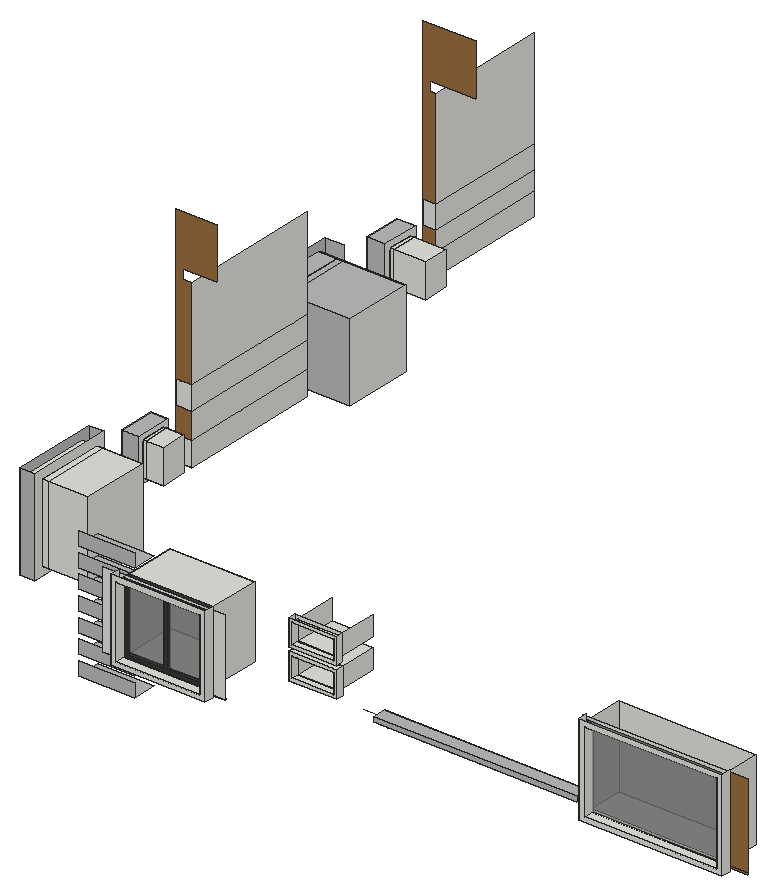
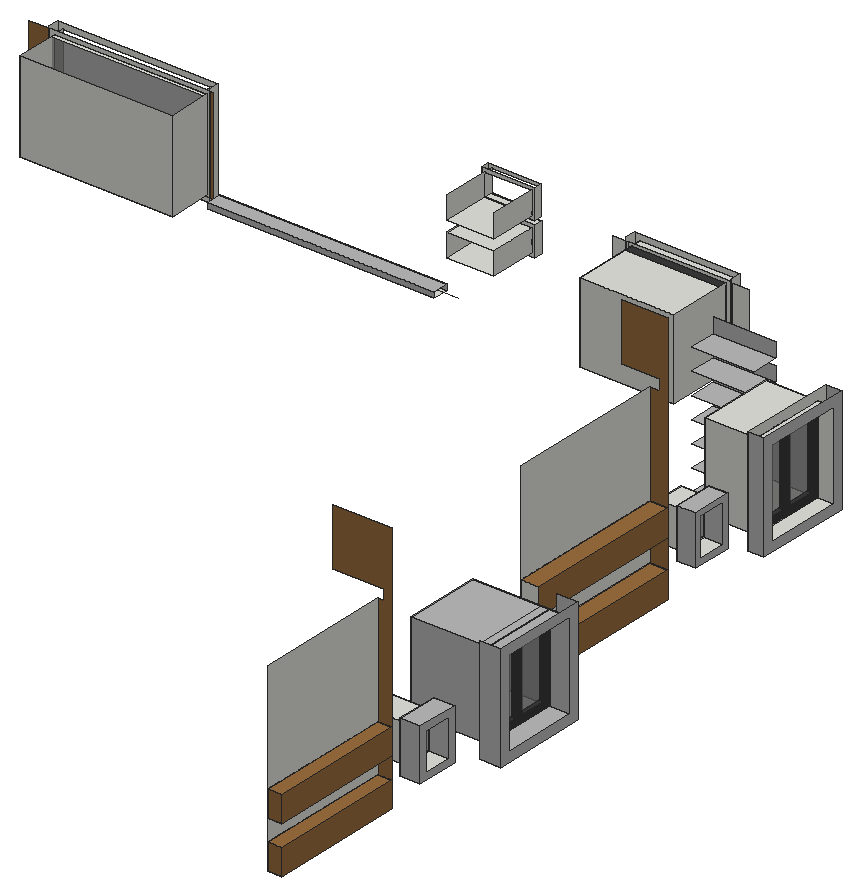
# SketchUp Ruby script. Lengths in inches.
U = 1.inch
M = Sketchup.active_model
def pt(a) = Geom::Point3d.new(a.map { |v| v * U })
def face(e, loops, mat)
  f = e.add_face(loops[0].map { |a| pt(a) })
  loops[1..].each { |l| e.add_face(l.map { |a| pt(a) }).erase! }
  f.material = f.back_material = mat if mat
  f
end
# faces: each face lists its corners as indices into pts; further lists are holes
def faces(e, pts, list, mat = nil) = list.each { |f| face(e, (f[0].is_a?(Array) ? f : [f]).map { |l| l.map { |i| pts[i] } }, mat) }
# xy, xz, yz: faces in a plane at the given z, y or x. An outline is a flat list of corners, or four numbers for a rectangle; further outlines are holes
def ring(l) = l.size == 4 ? [[l[0], l[1]], [l[2], l[1]], [l[2], l[3]], [l[0], l[3]]] : l.each_slice(2).to_a
def flat(e, list, mat, &to3) = list.each { |f| face(e, (f[0].is_a?(Array) ? f : [f]).map { |l| ring(l).map { |u, v| to3.(u, v) } }, mat) }
def xy(e, z, list, mat = nil) = flat(e, list, mat) { |x, y| [x, y, z] }
def xz(e, y, list, mat = nil) = flat(e, list, mat) { |x, z| [x, y, z] }
def yz(e, x, list, mat = nil) = flat(e, list, mat) { |y, z| [x, y, z] }
def lines(e, pts, list) = list.each { |a, b| e.add_line(pt(pts[a]), pt(pts[b])) }
# prism: a flat outline (further loops are holes) pulled along v
def prism(e, loops, v, mat = nil)
  f = face(e, loops, mat); d = Geom::Vector3d.new(v.map { |x| x * U })
  f.pushpull(f.normal.samedirection?(d) ? d.length : -d.length)
end
def box(e, o, s, mat = nil) = prism(e, [[o, [o[0] + s[0], o[1], o[2]], [o[0] + s[0], o[1] + s[1], o[2]], [o[0], o[1] + s[1], o[2]]]], [0, 0, s[2]], mat)
def at(x, y, z, deg = 0) = Geom::Transformation.translation(pt([x, y, z])) * Geom::Transformation.rotation(ORIGIN, Z_AXIS, deg.degrees)
def axes(o, x, y, z) = Geom::Transformation.new([*x, 0, *y, 0, *z, 0, *pt(o).to_a, 1])
def part(name) = M.definitions.add(name)
# library, detail: a bought-in or finely detailed component or shape, given as its bounding box
def library(name, o, s) = part(name).tap { |d| box(d.entities, o, s) }
def detail(e, o, s) = box(e.add_group.entities, o, s)
def put(e, d, t, mat = nil) = e.add_instance(d, t).tap { |i| i.material = mat if mat }
def group(e, t, mat = nil) = e.add_group.tap { |g| g.transformation = t; g.material = mat if mat }.entities
root = M.entities
M.materials.add("Generic").color = [155, 110, 63]
M.materials.add("Generic\#2").color = [186, 186, 186]
M.materials.add("[Color M07]").color = [58, 58, 58]
M.materials.add("[Translucent Glass Gray]").color = [127, 127, 127]
M.materials["[Translucent Glass Gray]"].alpha = 0.58
M.materials.add("[Translucent Glass Gray]1").color = [127, 127, 127]
M.materials["[Translucent Glass Gray]1"].alpha = 0.5
c1 = part("Group\#1")
xy(c1.entities,0,[[0,0,46.77,20.375]])
xz(c1.entities,0,[[0,0,46.77,11.0625]])
c2 = part("Group\#4")
xy(c2.entities,0,[[0,0,6,57.4375]],"[Color M07]")
xy(c2.entities,5.48,[[0,5.48,3,25.98],[0,31.46,3,51.96]],"[Color M07]")
xy(c2.entities,59.46,[[0,5.48,3,25.98],[0,31.46,3,51.96]],"[Color M07]")
xy(c2.entities,64.9375,[[0,0,6,57.4375]],"[Color M07]")
xz(c2.entities,0,[[0,0,6,64.9375]],"[Color M07]")
xz(c2.entities,5.48,[[0,5.48,3,59.46]],"[Color M07]")
xz(c2.entities,25.98,[[0,5.48,3,59.46]],"[Color M07]")
xz(c2.entities,31.46,[[0,5.48,3,59.46]],"[Color M07]")
xz(c2.entities,51.96,[[0,5.48,3,59.46]],"[Color M07]")
xz(c2.entities,57.4375,[[0,0,6,64.9375]],"[Color M07]")
yz(c2.entities,0,[[[0,0,57.4375,64.9375],[31.46,5.48,51.96,59.46],[5.48,5.48,25.98,59.46]]],"[Color M07]")
yz(c2.entities,3,[[5.48,5.48,25.98,59.46],[31.46,5.48,51.96,59.46]],"[Translucent Glass Gray]1")
yz(c2.entities,6,[[0,0,57.4375,64.9375]],"[Translucent Glass Gray]1")
c3 = part("Group\#3")
xy(c3.entities,0,[[0,0,70.4375,6]],"[Color M07]")
xy(c3.entities,2.83,[[2.83,0,33.8,3],[36.63,0,67.61,3]],"[Color M07]")
xy(c3.entities,56.73,[[2.83,0,33.8,3],[36.63,0,67.61,3]],"[Color M07]")
xy(c3.entities,59.5625,[[0,0,70.4375,6]],"[Color M07]")
xz(c3.entities,0,[[[0,0,70.4375,59.5625],[2.83,2.83,33.8,56.73],[36.63,2.83,67.61,56.73]]],"[Color M07]")
xz(c3.entities,3,[[2.83,2.83,33.8,56.73],[36.63,2.83,67.61,56.73]],"[Translucent Glass Gray]")
xz(c3.entities,6,[[0,0,70.4375,59.5625]],"[Translucent Glass Gray]")
yz(c3.entities,0,[[0,0,6,59.5625]],"[Color M07]")
yz(c3.entities,2.83,[[0,2.83,3,56.73]],"[Color M07]")
yz(c3.entities,33.8,[[0,2.83,3,56.73]],"[Color M07]")
yz(c3.entities,36.63,[[0,2.83,3,56.73]],"[Color M07]")
yz(c3.entities,67.61,[[0,2.83,3,56.73]],"[Color M07]")
yz(c3.entities,70.4375,[[0,0,6,59.5625]],"[Color M07]")
c4 = part("Group\#2")
xy(c4.entities,0,[[0,0,113.875,3]])
xy(c4.entities,67.5625,[[0,0,113.875,3]])
xz(c4.entities,0,[[0,0,113.875,67.5625]],"[Translucent Glass Gray]")
xz(c4.entities,3,[[0,0,113.875,67.5625]],"[Translucent Glass Gray]")
yz(c4.entities,0,[[0,0,3,67.5625]])
yz(c4.entities,113.875,[[0,0,3,67.5625]])
c5 = part("Group\#5")
xy(c5.entities,0,[[0,0,3,21.5625]])
xy(c5.entities,28.3125,[[0,0,3,21.5625]])
xz(c5.entities,0,[[0,0,3,28.3125]])
xz(c5.entities,21.5625,[[0,0,3,28.3125]])
yz(c5.entities,0,[[0,0,21.5625,28.3125]],"[Translucent Glass Gray]1")
yz(c5.entities,3,[[0,0,21.5625,28.3125]],"[Translucent Glass Gray]1")
xy(root,866.52,[[36.4375,161.95,48.5,234.18]],"Generic\#2")
xy(root,866.77,[[0,454.08,15.3125,525.8]],"Generic\#2")
xy(root,873.91,[[36.4375,169.34,48.5,226.78],[48.5,169.34,87,226.78]])
xy(root,873.91,[[0,461.22,72.5625,518.66]],"Generic\#2")
xy(root,877.875,[[170.35,89.25,249.19,97.25],[171.66,97.25,172.16,98],[247.01,97.25,247.51,98]])
xy(root,878.88,[[35,326.1875,48.5,446.1875]],"Generic")
xy(root,879.5,[[157.47,97.25,170.35,98],[249.19,97.25,259.3125,98]])
xy(root,879.52,[[538.69,116.625,658.46,124.5]])
xy(root,879.52,[[4.375,621.86,15.3125,724.5]],"Generic")
xy(root,880,[[157.47,97.25,170.35,98],[249.19,97.25,259.3125,98]])
xy(root,882.08,[[174.55,89.25,244.99,97.25],[174.55,97.25,244.99,145.8125]])
xy(root,883.72,[[543.83,116.625,654.26,124.5],[540.39,124.5,654.26,156.8125]])
xy(root,884.89,[[[359.25,127.31,528.75,138.74],[507.39,127.81,507.6,127.83,507.79,127.91,507.96,128.04,508.09,128.21,508.17,128.41,508.2,128.62,508.17,128.83,508.09,129.02,507.96,129.19,507.79,129.32,507.6,129.4,507.39,129.43,507.18,129.4,506.98,129.32,506.8125,129.19,506.68,129.02,506.6,128.83,506.57,128.62,506.6,128.41,506.68,128.21,506.8125,128.04,506.98,127.91,507.18,127.83],[501.32,127.81,501.53,127.83,501.73,127.91,501.9,128.04,502.03,128.21,502.11,128.41,502.14,128.62,502.11,128.83,502.03,129.02,501.9,129.19,501.73,129.32,501.53,129.4,501.32,129.43,501.11,129.4,500.92,129.32,500.75,129.19,500.62,129.02,500.54,128.83,500.51,128.62,500.54,128.41,500.62,128.21,500.75,128.04,500.92,127.91,501.11,127.83],[495.39,127.81,495.6,127.83,495.79,127.91,495.96,128.04,496.09,128.21,496.17,128.41,496.2,128.62,496.17,128.83,496.09,129.02,495.96,129.19,495.79,129.32,495.6,129.4,495.39,129.43,495.18,129.4,494.98,129.32,494.8125,129.19,494.68,129.02,494.6,128.83,494.57,128.62,494.6,128.41,494.68,128.21,494.8125,128.04,494.98,127.91,495.18,127.83],[489.89,127.81,490.1,127.83,490.29,127.91,490.46,128.04,490.59,128.21,490.67,128.41,490.7,128.62,490.67,128.83,490.59,129.02,490.46,129.19,490.29,129.32,490.1,129.4,489.89,129.43,489.68,129.4,489.48,129.32,489.3125,129.19,489.18,129.02,489.1,128.83,489.07,128.62,489.1,128.41,489.18,128.21,489.3125,128.04,489.48,127.91,489.68,127.83],[483.76,127.81,483.97,127.83,484.17,127.91,484.34,128.04,484.46,128.21,484.55,128.41,484.57,128.62,484.55,128.83,484.46,129.02,484.34,129.19,484.17,129.32,483.97,129.4,483.76,129.43,483.55,129.4,483.35,129.32,483.1875,129.19,483.06,129.02,482.98,128.83,482.95,128.62,482.98,128.41,483.06,128.21,483.1875,128.04,483.35,127.91,483.55,127.83],[477.76,127.81,477.97,127.83,478.17,127.91,478.34,128.04,478.46,128.21,478.55,128.41,478.57,128.62,478.55,128.83,478.46,129.02,478.34,129.19,478.17,129.32,477.97,129.4,477.76,129.43,477.55,129.4,477.35,129.32,477.1875,129.19,477.06,129.02,476.98,128.83,476.95,128.62,476.98,128.41,477.06,128.21,477.1875,128.04,477.35,127.91,477.55,127.83],[471.95,127.81,472.16,127.83,472.35,127.91,472.52,128.04,472.65,128.21,472.73,128.41,472.76,128.62,472.73,128.83,472.65,129.02,472.52,129.19,472.35,129.32,472.16,129.4,471.95,129.43,471.74,129.4,471.54,129.32,471.375,129.19,471.24,129.02,471.16,128.83,471.14,128.62,471.16,128.41,471.24,128.21,471.375,128.04,471.54,127.91,471.74,127.83],[465.76,127.81,465.97,127.83,466.17,127.91,466.34,128.04,466.46,128.21,466.55,128.41,466.57,128.62,466.55,128.83,466.46,129.02,466.34,129.19,466.17,129.32,465.97,129.4,465.76,129.43,465.55,129.4,465.35,129.32,465.1875,129.19,465.06,129.02,464.98,128.83,464.95,128.62,464.98,128.41,465.06,128.21,465.1875,128.04,465.35,127.91,465.55,127.83],[459.95,127.81,460.16,127.83,460.35,127.91,460.52,128.04,460.65,128.21,460.73,128.41,460.76,128.62,460.73,128.83,460.65,129.02,460.52,129.19,460.35,129.32,460.16,129.4,459.95,129.43,459.74,129.4,459.54,129.32,459.375,129.19,459.24,129.02,459.16,128.83,459.14,128.62,459.16,128.41,459.24,128.21,459.375,128.04,459.54,127.91,459.74,127.83],[453.89,127.81,454.1,127.83,454.29,127.91,454.46,128.04,454.59,128.21,454.67,128.41,454.7,128.62,454.67,128.83,454.59,129.02,454.46,129.19,454.29,129.32,454.1,129.4,453.89,129.43,453.68,129.4,453.48,129.32,453.3125,129.19,453.18,129.02,453.1,128.83,453.07,128.62,453.1,128.41,453.18,128.21,453.3125,128.04,453.48,127.91,453.68,127.83],[448.07,127.81,448.28,127.83,448.48,127.91,448.65,128.04,448.78,128.21,448.86,128.41,448.89,128.62,448.86,128.83,448.78,129.02,448.65,129.19,448.48,129.32,448.28,129.4,448.07,129.43,447.86,129.4,447.67,129.32,447.5,129.19,447.37,129.02,447.29,128.83,447.26,128.62,447.29,128.41,447.37,128.21,447.5,128.04,447.67,127.91,447.86,127.83],[442.01,127.81,442.22,127.83,442.42,127.91,442.59,128.04,442.71,128.21,442.8,128.41,442.82,128.62,442.8,128.83,442.71,129.02,442.59,129.19,442.42,129.32,442.22,129.4,442.01,129.43,441.8,129.4,441.6,129.32,441.4375,129.19,441.31,129.02,441.23,128.83,441.2,128.62,441.23,128.41,441.31,128.21,441.4375,128.04,441.6,127.91,441.8,127.83],[436.01,127.81,436.22,127.83,436.42,127.91,436.59,128.04,436.71,128.21,436.8,128.41,436.82,128.62,436.8,128.83,436.71,129.02,436.59,129.19,436.42,129.32,436.22,129.4,436.01,129.43,435.8,129.4,435.6,129.32,435.4375,129.19,435.31,129.02,435.23,128.83,435.2,128.62,435.23,128.41,435.31,128.21,435.4375,128.04,435.6,127.91,435.8,127.83],[430.2,127.81,430.41,127.83,430.6,127.91,430.77,128.04,430.9,128.21,430.98,128.41,431.01,128.62,430.98,128.83,430.9,129.02,430.77,129.19,430.6,129.32,430.41,129.4,430.2,129.43,429.99,129.4,429.79,129.32,429.625,129.19,429.49,129.02,429.41,128.83,429.39,128.62,429.41,128.41,429.49,128.21,429.625,128.04,429.79,127.91,429.99,127.83],[424.39,127.81,424.6,127.83,424.79,127.91,424.96,128.04,425.09,128.21,425.17,128.41,425.2,128.62,425.17,128.83,425.09,129.02,424.96,129.19,424.79,129.32,424.6,129.4,424.39,129.43,424.18,129.4,423.98,129.32,423.8125,129.19,423.68,129.02,423.6,128.83,423.57,128.62,423.6,128.41,423.68,128.21,423.8125,128.04,423.98,127.91,424.18,127.83],[418.45,127.81,418.66,127.83,418.85,127.91,419.02,128.04,419.15,128.21,419.23,128.41,419.26,128.62,419.23,128.83,419.15,129.02,419.02,129.19,418.85,129.32,418.66,129.4,418.45,129.43,418.24,129.4,418.04,129.32,417.875,129.19,417.74,129.02,417.66,128.83,417.64,128.62,417.66,128.41,417.74,128.21,417.875,128.04,418.04,127.91,418.24,127.83],[412.32,127.81,412.53,127.83,412.73,127.91,412.9,128.04,413.03,128.21,413.11,128.41,413.14,128.62,413.11,128.83,413.03,129.02,412.9,129.19,412.73,129.32,412.53,129.4,412.32,129.43,412.11,129.4,411.92,129.32,411.75,129.19,411.62,129.02,411.54,128.83,411.51,128.62,411.54,128.41,411.62,128.21,411.75,128.04,411.92,127.91,412.11,127.83],[406.39,127.81,406.6,127.83,406.79,127.91,406.96,128.04,407.09,128.21,407.17,128.41,407.2,128.62,407.17,128.83,407.09,129.02,406.96,129.19,406.79,129.32,406.6,129.4,406.39,129.43,406.18,129.4,405.98,129.32,405.8125,129.19,405.68,129.02,405.6,128.83,405.57,128.62,405.6,128.41,405.68,128.21,405.8125,128.04,405.98,127.91,406.18,127.83],[400.57,127.81,400.78,127.83,400.98,127.91,401.15,128.04,401.28,128.21,401.36,128.41,401.39,128.62,401.36,128.83,401.28,129.02,401.15,129.19,400.98,129.32,400.78,129.4,400.57,129.43,400.36,129.4,400.17,129.32,400,129.19,399.87,129.02,399.79,128.83,399.76,128.62,399.79,128.41,399.87,128.21,400,128.04,400.17,127.91,400.36,127.83],[394.76,127.81,394.97,127.83,395.17,127.91,395.34,128.04,395.46,128.21,395.55,128.41,395.57,128.62,395.55,128.83,395.46,129.02,395.34,129.19,395.17,129.32,394.97,129.4,394.76,129.43,394.55,129.4,394.35,129.32,394.1875,129.19,394.06,129.02,393.98,128.83,393.95,128.62,393.98,128.41,394.06,128.21,394.1875,128.04,394.35,127.91,394.55,127.83],[388.82,127.81,389.03,127.83,389.23,127.91,389.4,128.04,389.53,128.21,389.61,128.41,389.64,128.62,389.61,128.83,389.53,129.02,389.4,129.19,389.23,129.32,389.03,129.4,388.82,129.43,388.61,129.4,388.42,129.32,388.25,129.19,388.12,129.02,388.04,128.83,388.01,128.62,388.04,128.41,388.12,128.21,388.25,128.04,388.42,127.91,388.61,127.83],[382.76,127.81,382.97,127.83,383.17,127.91,383.34,128.04,383.46,128.21,383.55,128.41,383.57,128.62,383.55,128.83,383.46,129.02,383.34,129.19,383.17,129.32,382.97,129.4,382.76,129.43,382.55,129.4,382.35,129.32,382.1875,129.19,382.06,129.02,381.98,128.83,381.95,128.62,381.98,128.41,382.06,128.21,382.1875,128.04,382.35,127.91,382.55,127.83],[376.7,127.81,376.91,127.83,377.1,127.91,377.27,128.04,377.4,128.21,377.48,128.41,377.51,128.62,377.48,128.83,377.4,129.02,377.27,129.19,377.1,129.32,376.91,129.4,376.7,129.43,376.49,129.4,376.29,129.32,376.125,129.19,375.99,129.02,375.91,128.83,375.89,128.62,375.91,128.41,375.99,128.21,376.125,128.04,376.29,127.91,376.49,127.83],[365.01,127.81,365.22,127.83,365.42,127.91,365.59,128.04,365.71,128.21,365.8,128.41,365.82,128.62,365.8,128.83,365.71,129.02,365.59,129.19,365.42,129.32,365.22,129.4,365.01,129.43,364.8,129.4,364.6,129.32,364.4375,129.19,364.31,129.02,364.23,128.83,364.2,128.62,364.23,128.41,364.31,128.21,364.4375,128.04,364.6,127.91,364.8,127.83],[370.76,127.81,370.97,127.83,371.17,127.91,371.34,128.04,371.46,128.21,371.55,128.41,371.57,128.62,371.55,128.83,371.46,129.02,371.34,129.19,371.17,129.32,370.97,129.4,370.76,129.43,370.55,129.4,370.35,129.32,370.1875,129.19,370.06,129.02,369.98,128.83,369.95,128.62,369.98,128.41,370.06,128.21,370.1875,128.04,370.35,127.91,370.55,127.83]],[519.32,127.81,519.53,127.83,519.73,127.91,519.9,128.04,520.03,128.21,520.11,128.41,520.14,128.62,520.11,128.83,520.03,129.02,519.9,129.19,519.73,129.32,519.53,129.4,519.32,129.43,519.11,129.4,518.92,129.32,518.75,129.19,518.62,129.02,518.54,128.83,518.51,128.62,518.54,128.41,518.62,128.21,518.75,128.04,518.92,127.91,519.11,127.83]])
xy(root,886.75,[[513.45,127.81,513.66,127.83,513.85,127.91,514.02,128.04,514.15,128.21,514.23,128.41,514.26,128.62,514.23,128.83,514.15,129.02,514.02,129.19,513.85,129.32,513.66,129.4,513.45,129.43,513.24,129.4,513.04,129.32,512.875,129.19,512.74,129.02,512.66,128.83,512.64,128.62,512.66,128.41,512.74,128.21,512.875,128.04,513.04,127.91,513.24,127.83]])
xy(root,888.61,[[0,569.11,15.3125,600.97]],"Generic\#2")
xy(root,889.08,[[359.25,127.31,528.75,138.74]],"Generic\#2")
xy(root,889.11,[[34.5,270.92,48.5,300.91]],"Generic\#2")
xy(root,893.76,[[34.5,275.13,48.5,296.69],[48.5,275.13,65.625,296.69],[0,574.26,15.3125,595.82],[15.3125,574.26,44.75,595.82]])
xy(root,898.79,[[4.375,621.86,15.3125,724.5]],"Generic")
xy(root,898.89,[[35,326.1875,48.5,446.1875]],"Generic")
xy(root,912.72,[[312.22,97.5,352.19,103.5]])
xy(root,914.95,[[4.375,621.86,15.3125,724.5]],"Generic")
xy(root,915.33,[[314.83,97.5,349.58,103.5],[314.83,103.5,349.58,138.74]])
xy(root,920.5,[[35,326.1875,48.5,446.1875]],"Generic")
xy(root,922.07,[[34.5,275.13,48.5,296.69],[48.5,275.13,65.625,296.69],[0,574.26,15.3125,595.82],[15.3125,574.26,44.75,595.82]])
xy(root,926.29,[[34.5,270.92,48.5,300.91]],"Generic\#2")
xy(root,927.22,[[0,569.11,15.3125,600.97]],"Generic\#2")
xy(root,932.2,[[314.83,97.5,349.58,103.5],[314.83,103.5,349.58,138.74]])
xy(root,934.21,[[4.375,621.86,15.3125,724.5]],"Generic")
xy(root,934.81,[[312.22,97.5,352.19,103.5]])
xy(root,937.71,[[312.34,97.5,352.07,103.5]])
xy(root,938.85,[[36.4375,169.34,48.5,226.78],[48.5,169.34,87,226.78]])
xy(root,938.85,[[0,461.22,72.5625,518.66]],"Generic\#2")
xy(root,940.2,[[314.83,97.5,349.58,103.5],[314.83,103.5,349.58,138.74]])
xy(root,940.51,[[35,326.1875,48.5,446.1875]],"Generic")
xy(root,941.64,[[174.55,89.25,244.99,97.25],[174.55,97.25,244.99,145.8125]])
xz(root,89.25,[[[170.35,877.875,249.19,945.84],[174.55,882.08,244.99,941.64]]])
xz(root,97.25,[[170.35,877.875,171.66,879.5],[171.66,877.875,247.01,879.5],[247.01,877.875,249.19,879.5],[170.35,879.5,171.66,943.6875],[[171.66,879.5,247.01,943.6875],[174.55,882.08,244.99,941.64]],
  [247.01,879.5,249.19,943.6875],[157.47,880,170.35,943.1875],[249.19,880,259.3125,943.1875]])
xz(root,97.5,[[[312.22,912.72,352.19,934.81],[314.83,915.33,349.58,932.2]],[[312.34,937.71,352.07,959.57],[314.83,940.2,349.58,957.08]]])
xz(root,98,[[157.47,879.5,170.35,880],[249.19,879.5,259.3125,880]])
xz(root,103.5,[[[312.22,912.72,352.19,934.81],[314.83,915.33,349.58,932.2]],[[312.34,937.71,352.07,959.57],[314.83,940.2,349.58,957.08]]])
xz(root,116.625,[[[538.69,879.52,658.46,955.48],[543.83,883.72,654.26,951.29]]])
xz(root,124.5,[[538.69,879.52,658.46,882.5],[[538.69,882.5,658.46,954],[540.39,883.72,654.26,951.29]],[540.39,883.72,543.83,951.29]])
xz(root,124.5,[[535.75,882.5,538.69,954],[658.46,882.5,673.48,884],[658.46,884,673.48,954]],"Generic")
xz(root,127.31,[[359.25,884.89,528.75,889.08]],"Generic\#2")
xz(root,138.74,[[359.25,884.89,528.75,889.08]],"Generic\#2")
xz(root,145.8125,[[174.55,882.08,244.99,941.64]])
xz(root,156.8125,[[540.39,883.72,654.26,951.29]])
xz(root,161.95,[[36.4375,866.52,48.5,946.25]],"Generic\#2")
xz(root,169.34,[[36.4375,873.91,48.5,938.85],[48.5,873.91,87,938.85]])
xz(root,226.78,[[48.5,873.91,87,938.85]])
xz(root,226.78,[[36.4375,873.91,48.5,938.85]],"Generic\#2")
xz(root,234.18,[[36.4375,866.52,48.5,946.25]],"Generic\#2")
xz(root,270.92,[[34.5,889.11,48.5,926.29]],"Generic\#2")
xz(root,275.13,[[48.5,893.76,65.625,922.07]])
xz(root,275.13,[[34.5,893.76,48.5,922.07]],"Generic\#2")
xz(root,296.69,[[48.5,893.76,65.625,922.07]])
xz(root,296.69,[[34.5,893.76,48.5,922.07]],"Generic\#2")
xz(root,300.91,[[34.5,889.11,48.5,926.29]],"Generic\#2")
xz(root,326.1875,[[35,878.88,48.5,898.89],[35,920.5,48.5,940.51]])
xz(root,326.1875,[[35,898.89,48.5,920.5],[35,940.51,35,1067.5625,69,1067.5625,69,1024.6875,41,1024.6875,41,1016.8125,48.5,1016.8125,48.5,940.51]],"Generic")
xz(root,446.1875,[[35,878.88,48.5,898.89],[35,920.5,48.5,940.51]])
xz(root,454.08,[[0,866.77,15.3125,946]],"Generic\#2")
xz(root,461.22,[[0,873.91,72.5625,938.85]],"Generic\#2")
xz(root,518.66,[[0,873.91,72.5625,938.85]],"Generic\#2")
xz(root,525.8,[[0,866.77,15.3125,946]],"Generic\#2")
xz(root,569.11,[[0,888.61,15.3125,927.22]],"Generic\#2")
xz(root,574.26,[[15.3125,893.76,44.75,922.07]])
xz(root,574.26,[[0,893.76,15.3125,922.07]],"Generic\#2")
xz(root,595.82,[[15.3125,893.76,44.75,922.07]])
xz(root,595.82,[[0,893.76,15.3125,922.07]],"Generic\#2")
xz(root,600.97,[[0,888.61,15.3125,927.22]],"Generic\#2")
xz(root,621.86,[[4.375,879.52,15.3125,898.79],[4.375,914.95,15.3125,934.21]])
xz(root,621.86,[[4.375,898.79,15.3125,914.95],[4.375,934.21,4.375,1067.5625,48.5,1067.5625,48.5,1024.6875,10.5,1024.6875,10.5,1016.8125,15.3125,1016.8125,15.3125,934.21]],"Generic")
xz(root,724.5,[[4.375,879.52,15.3125,898.79],[4.375,914.95,15.3125,934.21]],"Generic")
yz(root,0,[[[454.08,866.77,525.8,946],[461.22,873.91,518.66,938.85]],[[569.11,888.61,600.97,927.22],[574.26,893.76,595.82,922.07]]],"Generic\#2")
yz(root,4.375,[[621.86,879.52,724.5,898.79],[621.86,914.95,724.5,934.21]],"Generic")
yz(root,15.3125,[[621.86,879.52,724.5,898.79],[[569.11,888.61,600.97,927.22],[574.26,893.76,595.82,922.07]],[621.86,898.79,724.5,914.95],[621.86,914.95,724.5,934.21],[621.86,934.21,724.5,1016.8125]])
yz(root,34.5,[[[270.92,889.11,300.91,926.29],[275.13,893.76,296.69,922.07]]],"Generic\#2")
yz(root,35,[[326.1875,878.88,446.1875,898.89],[326.1875,920.5,446.1875,940.51]],"Generic")
yz(root,36.4375,[[[161.95,866.52,234.18,946.25],[169.34,873.91,226.78,938.85]]],"Generic\#2")
yz(root,44.75,[[574.26,893.76,595.82,922.07]])
yz(root,48.5,[[[161.95,866.52,234.18,946.25],[169.34,873.91,226.78,938.85]],[326.1875,878.88,446.1875,898.89],[[270.92,889.11,300.91,926.29],[275.13,893.76,296.69,922.07]],[326.1875,898.89,446.1875,920.5],[326.1875,920.5,446.1875,940.51],
  [326.1875,940.51,446.1875,1016.8125]])
yz(root,65.625,[[275.13,893.76,296.69,922.07]])
yz(root,72.5625,[[461.22,873.91,518.66,938.85]])
yz(root,87,[[169.34,873.91,226.78,938.85]])
yz(root,170.35,[[89.25,877.875,97.25,945.84],[97.25,879.5,98,880]])
yz(root,174.55,[[89.25,882.08,97.25,941.64],[97.25,882.08,145.8125,941.64]])
yz(root,244.99,[[89.25,882.08,97.25,941.64],[97.25,882.08,145.8125,941.64]])
yz(root,249.19,[[89.25,877.875,97.25,945.84],[97.25,879.5,98,880]])
yz(root,312.22,[[97.5,912.72,103.5,934.81]])
yz(root,312.34,[[97.5,937.71,103.5,959.57]])
yz(root,314.83,[[97.5,915.33,103.5,932.2],[103.5,915.33,138.74,932.2],[97.5,940.2,103.5,957.08],[103.5,940.2,138.74,957.08]])
yz(root,349.58,[[97.5,915.33,103.5,932.2],[103.5,915.33,138.74,932.2],[97.5,940.2,103.5,957.08],[103.5,940.2,138.74,957.08]])
yz(root,352.07,[[97.5,937.71,103.5,959.57]])
yz(root,352.19,[[97.5,912.72,103.5,934.81]])
yz(root,538.69,[[116.625,879.52,124.5,955.48]])
yz(root,540.39,[[124.5,883.72,156.8125,951.29]])
yz(root,543.83,[[116.625,883.72,124.5,951.29]])
yz(root,654.26,[[116.625,883.72,124.5,951.29],[124.5,883.72,156.8125,951.29]])
yz(root,658.46,[[116.625,879.52,124.5,955.48]])
p = [[528.75,133.4,887.11],[345.9375,133.4,887.11]]
lines(root,p,[[0,1]])
put(root,c1,at(110.7,130.3125,831),"Generic\#2")
put(root,c1,at(110.7,130.3125,847.1875),"Generic\#2")
put(root,c1,at(110.7,130.3125,863.375),"Generic\#2")
put(root,c2,at(48.5,169.34,873.91))
put(root,c2,at(15.3125,461.22,873.91),"Generic\#2")
put(root,c1,at(110.7,130.3125,879.5625),"Generic\#2")
put(root,c3,at(174.55,97.25,882.08))
put(root,c4,at(540.39,124.5,883.72))
put(root,c5,at(48.5,275.13,893.76))
put(root,c5,at(15.3125,574.26,893.76))
put(root,c1,at(110.7,130.3125,895.75),"Generic\#2")
put(root,c1,at(110.7,130.3125,911.9375),"Generic\#2")
put(root,c1,at(110.7,130.3125,928.125),"Generic\#2")
